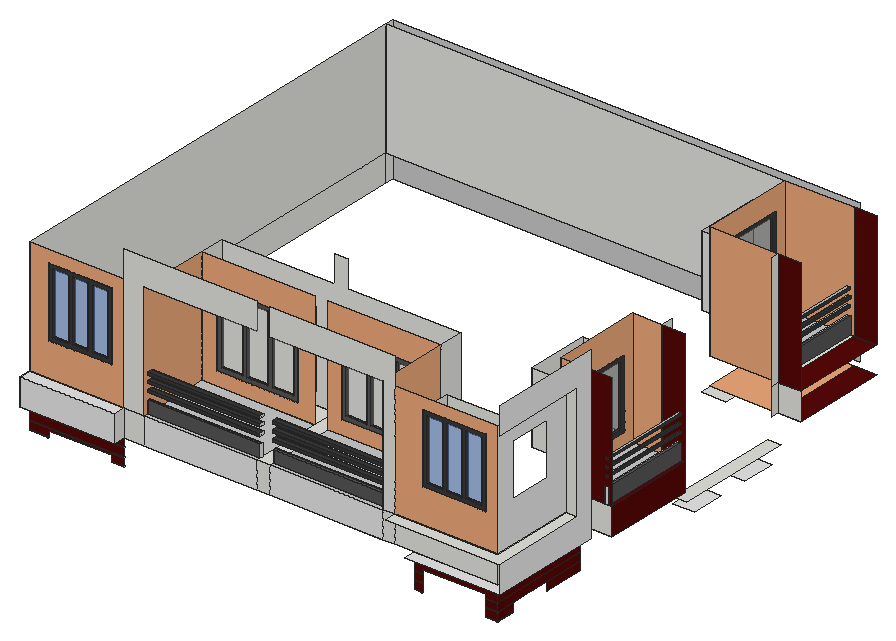
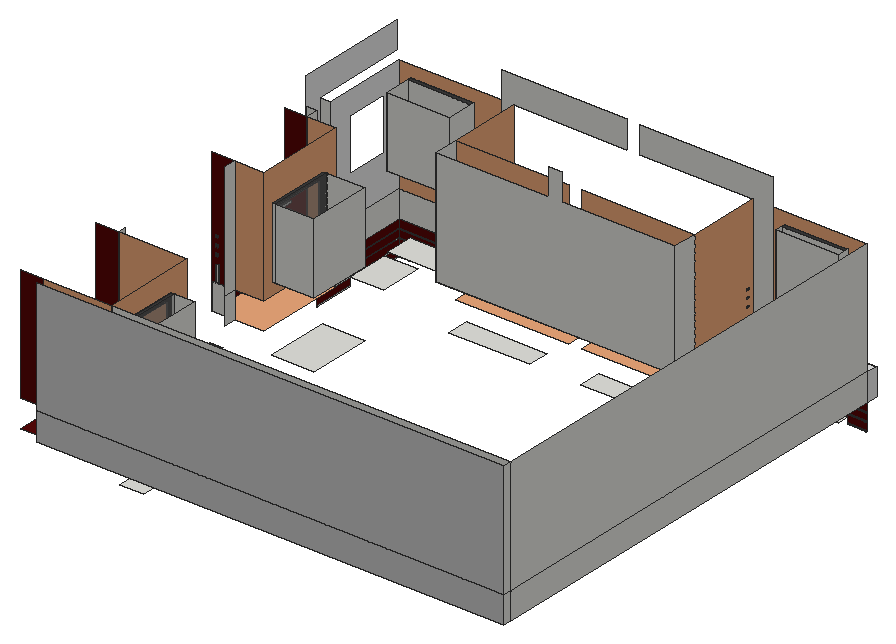
# SketchUp Ruby script. Lengths in inches.
U = 1.inch
M = Sketchup.active_model
def pt(a) = Geom::Point3d.new(a.map { |v| v * U })
def face(e, loops, mat)
  f = e.add_face(loops[0].map { |a| pt(a) })
  loops[1..].each { |l| e.add_face(l.map { |a| pt(a) }).erase! }
  f.material = f.back_material = mat if mat
  f
end
# faces: each face lists its corners as indices into pts; further lists are holes
def faces(e, pts, list, mat = nil) = list.each { |f| face(e, (f[0].is_a?(Array) ? f : [f]).map { |l| l.map { |i| pts[i] } }, mat) }
# xy, xz, yz: faces in a plane at the given z, y or x. An outline is a flat list of corners, or four numbers for a rectangle; further outlines are holes
def ring(l) = l.size == 4 ? [[l[0], l[1]], [l[2], l[1]], [l[2], l[3]], [l[0], l[3]]] : l.each_slice(2).to_a
def flat(e, list, mat, &to3) = list.each { |f| face(e, (f[0].is_a?(Array) ? f : [f]).map { |l| ring(l).map { |u, v| to3.(u, v) } }, mat) }
def xy(e, z, list, mat = nil) = flat(e, list, mat) { |x, y| [x, y, z] }
def xz(e, y, list, mat = nil) = flat(e, list, mat) { |x, z| [x, y, z] }
def yz(e, x, list, mat = nil) = flat(e, list, mat) { |y, z| [x, y, z] }
def lines(e, pts, list) = list.each { |a, b| e.add_line(pt(pts[a]), pt(pts[b])) }
# prism: a flat outline (further loops are holes) pulled along v
def prism(e, loops, v, mat = nil)
  f = face(e, loops, mat); d = Geom::Vector3d.new(v.map { |x| x * U })
  f.pushpull(f.normal.samedirection?(d) ? d.length : -d.length)
end
def box(e, o, s, mat = nil) = prism(e, [[o, [o[0] + s[0], o[1], o[2]], [o[0] + s[0], o[1] + s[1], o[2]], [o[0], o[1] + s[1], o[2]]]], [0, 0, s[2]], mat)
def at(x, y, z, deg = 0) = Geom::Transformation.translation(pt([x, y, z])) * Geom::Transformation.rotation(ORIGIN, Z_AXIS, deg.degrees)
def axes(o, x, y, z) = Geom::Transformation.new([*x, 0, *y, 0, *z, 0, *pt(o).to_a, 1])
def part(name) = M.definitions.add(name)
# library, detail: a bought-in or finely detailed component or shape, given as its bounding box
def library(name, o, s) = part(name).tap { |d| box(d.entities, o, s) }
def detail(e, o, s) = box(e.add_group.entities, o, s)
def put(e, d, t, mat = nil) = e.add_instance(d, t).tap { |i| i.material = mat if mat }
def group(e, t, mat = nil) = e.add_group.tap { |g| g.transformation = t; g.material = mat if mat }.entities
root = M.entities
M.materials.add("Generic").color = [86, 8, 8]
M.materials.add("Generic\#1").color = [236, 168, 122]
M.materials.add("Generic\#4").color = [201, 201, 201]
M.materials.add("Generic\#5").color = [230, 230, 230]
M.materials.add("[Color M06]").color = [86, 86, 86]
M.materials.add("[Color M07]").color = [58, 58, 58]
M.materials.add("[Mirror 02]1").color = [226, 226, 226]
M.materials["[Mirror 02]1"].alpha = 0.26
M.materials.add("[Translucent Glass Blue]").color = [100, 149, 237]
M.materials["[Translucent Glass Blue]"].alpha = 0.5
M.materials.add("[Translucent Glass Gray]").color = [127, 127, 127]
M.materials["[Translucent Glass Gray]"].alpha = 0.35
c1 = library("Tlon Light 450 Ceiling 152 006",[-8.86,-8.86,-3.78],[17.72,17.72,3.56])
c2 = part("Group\#5")
xy(c2.entities,0,[[0,0,6,92.0625]],"[Color M07]")
xy(c2.entities,6.58,[[3,6.58,6,85.48]],"[Color M07]")
xy(c2.entities,96.73,[[3,6.58,6,85.48]],"[Color M07]")
xy(c2.entities,103.3125,[[0,0,6,92.0625]],"[Color M07]")
xz(c2.entities,0,[[0,0,6,103.3125]],"[Color M07]")
xz(c2.entities,6.58,[[3,6.58,6,96.73]],"[Color M07]")
xz(c2.entities,85.48,[[3,6.58,6,96.73]],"[Color M07]")
xz(c2.entities,92.0625,[[0,0,6,103.3125]],"[Color M07]")
yz(c2.entities,0,[[0,0,92.0625,103.3125]],"[Translucent Glass Gray]")
yz(c2.entities,3,[[6.58,6.58,85.48,96.73]],"[Translucent Glass Gray]")
yz(c2.entities,6,[[[0,0,92.0625,103.3125],[6.58,6.58,85.48,96.73]]],"[Color M07]")
c3 = part("Group\#4")
xy(c3.entities,0,[[0,0,117.75,6]],"[Color M06]")
xy(c3.entities,6.37,[[6.37,0,37.125,3],[43.5,0,74.25,3],[80.625,0,111.38,3]],"[Color M06]")
xy(c3.entities,103.75,[[6.37,0,37.125,3],[43.5,0,74.25,3],[80.625,0,111.38,3]],"[Color M06]")
xy(c3.entities,110.125,[[0,0,117.75,6]],"[Color M06]")
xz(c3.entities,0,[[[0,0,117.75,110.125],[6.37,6.37,37.125,103.75],[80.625,6.37,111.38,103.75],[43.5,6.37,74.25,103.75]]],"[Color M06]")
xz(c3.entities,3,[[6.37,6.37,37.125,103.75],[43.5,6.37,74.25,103.75],[80.625,6.37,111.38,103.75]],"[Mirror 02]1")
xz(c3.entities,6,[[0,0,117.75,110.125]])
yz(c3.entities,0,[[0,0,6,110.125]],"[Color M06]")
yz(c3.entities,6.37,[[0,6.37,3,103.75]],"[Color M06]")
yz(c3.entities,37.125,[[0,6.37,3,103.75]],"[Color M06]")
yz(c3.entities,43.5,[[0,6.37,3,103.75]],"[Color M06]")
yz(c3.entities,74.25,[[0,6.37,3,103.75]],"[Color M06]")
yz(c3.entities,80.625,[[0,6.37,3,103.75]],"[Color M06]")
yz(c3.entities,111.38,[[0,6.37,3,103.75]],"[Color M06]")
yz(c3.entities,117.75,[[0,0,6,110.125]],"[Color M06]")
c4 = part("Group\#2")
xy(c4.entities,0,[[0,0,91.6875,6]],"[Color M07]")
xy(c4.entities,6.1,[[6.1,0,28.53,3],[34.63,0,57.06,3],[63.16,0,85.59,3]],"[Color M07]")
xy(c4.entities,95.34,[[6.1,0,28.53,3],[34.63,0,57.06,3],[63.16,0,85.59,3]],"[Color M07]")
xy(c4.entities,101.4375,[[0,0,91.6875,6]],"[Color M07]")
xz(c4.entities,0,[[[0,0,91.6875,101.4375],[34.63,6.1,57.06,95.34],[63.16,6.1,85.59,95.34],[6.1,6.1,28.53,95.34]]],"[Color M07]")
xz(c4.entities,3,[[6.1,6.1,28.53,95.34],[34.63,6.1,57.06,95.34],[63.16,6.1,85.59,95.34]],"[Translucent Glass Blue]")
xz(c4.entities,6,[[0,0,91.6875,101.4375]])
yz(c4.entities,0,[[0,0,6,101.4375]],"[Color M07]")
yz(c4.entities,6.1,[[0,6.1,3,95.34]],"[Color M07]")
yz(c4.entities,28.53,[[0,6.1,3,95.34]],"[Color M07]")
yz(c4.entities,34.63,[[0,6.1,3,95.34]],"[Color M07]")
yz(c4.entities,57.06,[[0,6.1,3,95.34]],"[Color M07]")
yz(c4.entities,63.16,[[0,6.1,3,95.34]],"[Color M07]")
yz(c4.entities,85.59,[[0,6.1,3,95.34]],"[Color M07]")
yz(c4.entities,91.6875,[[0,0,6,101.4375]],"[Color M07]")
xy(root,741.1,[[577.6875,113.625,589.83,113.92],[681.51,113.625,698.4375,113.92],[698.14,113.92,698.4375,141.33]])
xy(root,741.23,[[698.14,204.02,698.4375,263.625]])
xy(root,742.1,[[577.6875,113.625,589.83,113.92],[681.51,113.625,698.14,113.92]])
xy(root,742.11,[[698.14,113.625,698.4375,141.33]])
xy(root,742.23,[[698.14,204.02,698.4375,263.625]])
xy(root,743.55,[[685.875,449.87,717.1875,498.18],[685.875,541.87,717.1875,590.18]],"Generic\#5")
xy(root,751.9375,[[16.6875,113.625,44.83,113.625,44.83,113.93,16.6875,113.92],[136.51,113.625,154.5,113.625,154.5,113.92,136.51,113.93]])
xy(root,752.29,[[594.5625,306.16,656.0625,398.23]])
xy(root,752.9375,[[16.6875,113.625,16.6875,113.92,44.83,113.93,44.83,113.625],[136.51,113.625,136.51,113.93,154.5,113.92,154.5,113.625]])
xy(root,753.05,[[577.6875,113.625,589.83,113.625,589.83,113.93,577.6875,113.92],[681.51,113.625,698.4375,113.625,698.4375,113.92,698.14,113.92,681.51,113.93],[698.14,113.92,698.4375,141.33]])
xy(root,753.13,[[698.14,204.02,698.4375,263.625]])
xy(root,754.05,[[577.6875,113.625,577.6875,113.92,589.83,113.93,589.83,113.625],[681.51,113.625,681.51,113.93,698.14,113.92,698.4375,113.92,698.4375,113.625],[698.14,113.92,698.4375,141.33]])
xy(root,754.13,[[698.14,204.02,698.4375,263.625]])
xy(root,754.24,[[648.625,141.33,698.4375,204.02]])
xy(root,755.96,[[563.75,654.65,598.75,746.71]])
xy(root,761.05,[[44.83,113.625,136.51,130.0625]])
xy(root,762.91,[[698.4375,434.68,717.1875,606.05]])
xy(root,764.4375,[[16.6875,113.625,154.5,113.92]])
xy(root,764.99,[[577.6875,113.625,589.83,113.625,589.83,113.93,577.6875,113.92],[681.51,113.625,698.4375,113.625,698.4375,113.92,681.51,113.93]])
xy(root,765.04,[[698.14,113.92,698.4375,263.625]])
xy(root,765.4375,[[16.6875,113.625,154.5,113.92]])
xy(root,765.99,[[577.6875,113.625,577.6875,113.92,589.83,113.93,589.83,113.625],[681.51,113.625,681.51,113.93,698.14,113.92,698.14,113.625]])
xy(root,766.04,[[698.14,113.625,698.4375,263.625]])
xy(root,766.34,[[205.11,219.4375,322.86,251.5625],[397.99,219.4375,515.74,251.5625]])
xy(root,771.36,[[589.83,113.625,681.51,156.125]])
xy(root,776.9375,[[16.6875,113.625,154.5,113.92],[577.6875,113.625,698.4375,113.92],[698.14,113.92,698.4375,263.625]])
xy(root,777.9375,[[16.6875,113.625,154.5,113.92],[577.6875,113.625,698.4375,113.92],[698.14,113.92,698.4375,263.625]])
xy(root,789.9375,[[698.4375,624.8125,731.4375,762.8125]],"Generic")
xy(root,789.9375,[[183.5625,113.625,347.9375,219.4375],[367.1875,113.625,531.5625,219.4375],[656.0625,281.625,731.4375,413.625],[598.75,624.8125,698.4375,762.8125]],"Generic\#1")
xy(root,789.9375,[[16.6875,96.5625,154.5,113.625],[577.6875,96.5625,577.6875,113.625,698.4375,113.625,698.4375,263.625,715.125,263.625,715.125,96.5625]],"Generic\#5")
xy(root,829.25,[[549.5625,96.5625,715.125,96.5625,715.125,238.3125,698.4375,238.3125,698.4375,113.625,549.5625,113.625],[347.9375,113.625,367.1875,255],[183.5625,119.625,347.9375,123.625],[367.1875,119.625,531.5625,123.625],[183.5625,219.4375,347.9375,255],
  [367.1875,219.4375,531.5625,255],[721.25,281.625,726.125,413.625],[689.125,624.8125,693.625,762.8125],[693.625,624.8125,698.4375,762.8125]])
xy(root,829.25,[[726.125,281.625,731.4375,413.625],[698.4375,624.8125,731.4375,762.8125]],"Generic")
xy(root,829.25,[[183.5625,113.625,347.9375,119.625],[367.1875,113.625,531.5625,119.625],[183.5625,123.625,347.9375,219.4375],[367.1875,123.625,531.5625,219.4375],[656.0625,281.625,721.25,413.625],
  [598.75,624.8125,689.125,762.8125]],"Generic\#4")
xy(root,829.25,[[16.6875,96.5625,154.5,113.625]],"Generic\#5")
xy(root,847.25,[[183.5625,119.625,347.9375,123.625],[367.1875,119.625,531.5625,123.625]],"[Color M06]")
xy(root,848.17,[[594.5625,306.16,656.0625,398.23]])
xy(root,849.15,[[205.11,219.4375,322.86,251.5625],[386.36,219.4375,504.11,251.5625]])
xy(root,853.25,[[721.25,281.625,726.125,413.625],[689.125,624.8125,693.625,762.8125]],"[Color M06]")
xy(root,857.82,[[367.1875,118.5,531.5625,125.9375]],"[Color M07]")
xy(root,857.85,[[183.5625,118.5,347.9375,125.9375]],"[Color M07]")
xy(root,861.63,[[367.1875,118.5,531.5625,125.9375]],"[Color M07]")
xy(root,861.67,[[183.5625,118.5,347.9375,125.9375]],"[Color M07]")
xy(root,863.09,[[563.75,654.65,598.75,746.71]])
xy(root,864.125,[[688.99,624.8125,693.18,762.8125]],"[Color M07]")
xy(root,864.35,[[722.32,281.625,725.7,413.625]],"[Color M07]")
xy(root,867.4375,[[688.99,624.8125,693.18,762.8125]],"[Color M07]")
xy(root,867.48,[[722.32,281.625,725.7,413.625]],"[Color M07]")
xy(root,869.58,[[367.1875,118.5,531.5625,125.9375]],"[Color M07]")
xy(root,869.85,[[183.5625,118.5,347.9375,125.9375]],"[Color M07]")
xy(root,873.39,[[367.1875,118.5,531.5625,125.9375]],"[Color M07]")
xy(root,873.67,[[183.5625,118.5,347.9375,125.9375]],"[Color M07]")
xy(root,876.125,[[689.37,624.8125,693.56,762.8125]],"[Color M07]")
xy(root,876.22,[[722.32,281.625,725.7,413.625]],"[Color M07]")
xy(root,878.93,[[44.83,113.625,136.51,130.0625],[589.83,113.625,681.51,158.0625]])
xy(root,879.34,[[722.32,281.625,725.7,413.625]],"[Color M07]")
xy(root,879.4375,[[689.37,624.8125,693.56,762.8125]],"[Color M07]")
xy(root,880.92,[[183.5625,118.5,347.9375,125.9375]],"[Color M07]")
xy(root,881.34,[[367.1875,118.5,531.5625,125.9375]],"[Color M07]")
xy(root,884.73,[[183.5625,118.5,347.9375,125.9375]],"[Color M07]")
xy(root,885.15,[[367.1875,118.5,531.5625,125.9375]],"[Color M07]")
xy(root,888.125,[[688.93,624.8125,693.12,762.8125]],"[Color M07]")
xy(root,888.22,[[722.32,281.625,725.7,413.625]],"[Color M07]")
xz(root,96.5625,[[16.6875,789.9375,154.5,829.25]],"Generic\#5")
xz(root,113.625,[[16.6875,789.9375,154.5,829.25],[154.5,789.9375,183.4375,829.25],[347.9375,789.9375,367.1875,829.25],[531.6875,789.9375,549.5625,829.25],[549.5625,789.9375,698.4375,829.25],
  [154.5,829.25,154.5,1036.5625,347.9375,1036.5625,347.9375,997.25,183.4375,997.25,183.4375,829.25],[183.4375,829.25,183.5625,997.25],[531.6875,829.25,531.6875,997.25,367.1875,997.25,367.1875,1036.5625,549.5625,1036.5625,549.5625,829.25],[531.5625,829.25,531.6875,997.25]])
xz(root,113.625,[[577.6875,742.1,589.83,753.05],[681.51,742.1,698.14,742.1,698.14,742.11,698.4375,742.11,698.4375,753.05,681.51,753.05],[16.6875,752.9375,44.83,752.9375,44.83,761.05,136.51,761.05,136.51,752.9375,154.5,752.9375,154.5,764.4375,16.6875,764.4375],[577.6875,754.05,589.83,764.99],[681.51,754.05,698.4375,764.99],
  [16.6875,765.4375,154.5,776.9375],[577.6875,765.99,589.83,765.99,589.83,771.36,681.51,771.36,681.51,765.99,698.14,765.99,698.14,766.04,698.4375,766.04,698.4375,776.9375,577.6875,776.9375],[16.6875,777.9375,154.5,789.9375],[577.6875,777.9375,698.4375,789.9375]],"Generic")
xz(root,113.625,[[[16.6875,829.25,154.5,997.25],[44.83,878.93,136.51,980.36]],[[549.5625,829.25,698.4375,997.25],[589.83,878.93,681.51,980.36]]],"Generic\#1")
xz(root,113.625,[[183.4375,789.9375,347.9375,829.25],[367.1875,789.9375,531.6875,829.25]],"Generic\#5")
xz(root,113.92,[[577.6875,741.1,589.83,742.1],[681.51,741.1,698.14,742.1],[16.6875,764.4375,154.5,765.4375],[16.6875,776.9375,154.5,777.9375],[577.6875,776.9375,698.14,777.9375]])
xz(root,118.5,[[367.1875,857.82,531.5625,861.63],[183.5625,857.85,347.9375,861.67],[367.1875,869.58,531.5625,873.39],[183.5625,869.85,347.9375,873.67],[183.5625,880.92,347.9375,884.73],
  [367.1875,881.34,531.5625,885.15]],"[Color M07]")
xz(root,119.625,[[183.5625,829.25,347.9375,847.25],[367.1875,829.25,531.5625,847.25]],"[Color M06]")
xz(root,123.625,[[183.5625,829.25,347.9375,847.25],[367.1875,829.25,531.5625,847.25]])
xz(root,125.9375,[[367.1875,857.82,531.5625,861.63],[183.5625,857.85,347.9375,861.67],[367.1875,869.58,531.5625,873.39],[183.5625,869.85,347.9375,873.67],[183.5625,880.92,347.9375,884.73],
  [367.1875,881.34,531.5625,885.15]])
xz(root,130.0625,[[44.83,878.93,136.51,980.36]])
xz(root,158.0625,[[589.83,878.93,681.51,980.36]])
xz(root,219.4375,[[[183.5625,829.25,347.9375,997.25],[205.11,849.15,322.86,959.27]],[[367.1875,829.25,531.5625,997.25],[386.36,849.15,504.11,959.27]]],"Generic\#1")
xz(root,238.3125,[[698.4375,829.25,715.125,997.25]])
xz(root,251.5625,[[205.11,849.15,322.86,959.27],[386.36,849.15,504.11,959.27]])
xz(root,255,[[183.5625,829.25,531.5625,829.25,531.5625,997.25,367.1875,997.25,367.1875,1036.5625,347.9375,1036.5625,347.9375,997.25,183.5625,997.25]])
xz(root,263.625,[[698.14,741.23,698.4375,742.23],[698.14,753.13,698.4375,754.13],[698.14,765.04,698.4375,766.04],[698.14,776.9375,698.4375,777.9375],[698.4375,789.9375,715.125,829.25],
  [698.4375,829.25,715.125,997.25]])
xz(root,281.625,[[698.4375,789.9375,731.4375,829.25],[721.25,829.25,726.125,853.25]])
xz(root,281.625,[[[698.4375,829.25,698.4375,997.25,731.4375,997.25,731.4375,829.25,726.125,829.25,726.125,853.25,721.25,853.25,721.25,829.25],[722.32,888.22,725.7,891.34],[722.32,876.22,725.7,879.34],[722.32,864.35,725.7,867.48]]],"Generic")
xz(root,281.625,[[656.0625,829.25,698.4375,997.25]],"Generic\#1")
xz(root,306.16,[[594.5625,848.17,656.0625,951.48]])
xz(root,398.23,[[594.5625,848.17,656.0625,951.48]])
xz(root,413.625,[[698.4375,789.9375,731.4375,829.25],[721.25,829.25,726.125,853.25],[722.32,864.35,725.7,867.48],[722.32,876.22,725.7,879.34],[722.32,888.22,725.7,891.34]])
xz(root,413.625,[[[698.4375,829.25,721.25,829.25,721.25,853.25,726.125,853.25,726.125,829.25,731.4375,829.25,731.4375,997.25,698.4375,997.25],[722.32,864.35,725.7,867.48],[722.32,876.22,725.7,879.34],[722.32,888.22,725.7,891.34]]],"Generic")
xz(root,413.625,[[656.0625,829.25,698.4375,997.25]],"Generic\#1")
xz(root,624.8125,[[698.4375,789.9375,731.4375,829.25],[689.125,829.25,693.625,853.25]])
xz(root,624.8125,[[698.4375,829.25,731.4375,997.25]],"Generic")
xz(root,624.8125,[[[598.75,829.25,598.75,997.25,698.4375,997.25,698.4375,829.25,693.625,829.25,693.625,853.25,689.125,853.25,689.125,829.25],[688.93,888.125,693.12,891.4375],[689.37,876.125,693.56,879.4375],[688.99,864.125,693.18,867.4375]]],"Generic\#1")
xz(root,654.65,[[563.75,863.09,598.75,966.4]])
xz(root,746.71,[[563.75,863.09,598.75,966.4]])
xz(root,762.8125,[[16.6875,829.25,598.75,997.25],[689.125,829.25,693.625,853.25],[688.99,864.125,693.18,867.4375],[689.37,876.125,693.56,879.4375],[688.93,888.125,693.12,891.4375]])
xz(root,762.8125,[[698.4375,829.25,731.4375,997.25]],"Generic")
xz(root,762.8125,[[[598.75,829.25,689.125,829.25,689.125,853.25,693.625,853.25,693.625,829.25,698.4375,829.25,698.4375,997.25,598.75,997.25],[688.99,864.125,693.18,867.4375],[689.37,876.125,693.56,879.4375],[688.93,888.125,693.12,891.4375]]],"Generic\#1")
xz(root,774.8125,[[16.6875,789.9375,698.4375,829.25],[16.6875,829.25,698.4375,997.25]],"Generic\#4")
yz(root,16.6875,[[113.625,789.9375,762.8125,829.25],[762.8125,789.9375,774.8125,829.25],[113.625,829.25,762.8125,997.25],[762.8125,829.25,774.8125,997.25]])
yz(root,16.6875,[[96.5625,789.9375,113.625,829.25]],"Generic\#5")
yz(root,44.83,[[113.625,878.93,130.0625,980.36]])
yz(root,136.51,[[113.625,878.93,130.0625,980.36]])
yz(root,154.5,[[113.625,751.9375,113.92,752.9375],[113.625,764.4375,113.92,765.4375],[113.625,776.9375,113.92,777.9375],[96.5625,789.9375,113.625,829.25]])
yz(root,183.5625,[[119.625,829.25,123.625,847.25],[219.4375,829.25,255,997.25]])
yz(root,183.5625,[[[113.625,829.25,119.625,829.25,119.625,847.25,123.625,847.25,123.625,829.25,219.4375,829.25,219.4375,997.25,113.625,997.25],[118.5,880.92,125.9375,884.73],[118.5,869.85,125.9375,873.67],[118.5,857.85,125.9375,861.67]]],"Generic\#1")
yz(root,205.11,[[219.4375,849.15,251.5625,959.27]])
yz(root,322.86,[[219.4375,849.15,251.5625,959.27]])
yz(root,347.9375,[[119.625,829.25,123.625,847.25],[118.5,857.85,125.9375,861.67],[118.5,869.85,125.9375,873.67],[118.5,880.92,125.9375,884.73]])
yz(root,367.1875,[[119.625,829.25,123.625,847.25]])
yz(root,386.36,[[219.4375,849.15,251.5625,959.27]])
yz(root,504.11,[[219.4375,849.15,251.5625,959.27]])
yz(root,531.5625,[[119.625,829.25,123.625,847.25],[219.4375,829.25,255,997.25],[118.5,857.82,125.9375,861.63],[118.5,869.58,125.9375,873.39],[118.5,881.34,125.9375,885.15]])
yz(root,531.5625,[[[113.625,829.25,113.625,997.25,219.4375,997.25,219.4375,829.25,123.625,829.25,123.625,847.25,119.625,847.25,119.625,829.25],[118.5,881.34,125.9375,885.15],[118.5,869.58,125.9375,873.39],[118.5,857.82,125.9375,861.63]]],"Generic\#1")
yz(root,563.75,[[654.65,863.09,746.71,966.4]])
yz(root,577.6875,[[113.625,741.1,113.92,742.1],[113.625,753.05,113.92,754.05],[113.625,764.99,113.92,765.99],[113.625,776.9375,113.92,777.9375]])
yz(root,589.83,[[113.625,878.93,158.0625,980.36]])
yz(root,594.5625,[[306.16,848.17,398.23,951.48]])
yz(root,598.75,[[[624.8125,829.25,762.8125,997.25],[654.65,863.09,746.71,966.4]]],"Generic\#1")
yz(root,656.0625,[[[281.625,829.25,413.625,997.25],[306.16,848.17,398.23,951.48]]],"Generic\#1")
yz(root,681.51,[[113.625,878.93,158.0625,980.36]])
yz(root,688.93,[[624.8125,888.125,762.8125,891.4375]])
yz(root,688.99,[[624.8125,864.125,762.8125,867.4375]])
yz(root,689.125,[[624.8125,829.25,762.8125,853.25]])
yz(root,689.37,[[624.8125,876.125,762.8125,879.4375]])
yz(root,693.12,[[624.8125,888.125,762.8125,891.4375]],"[Color M07]")
yz(root,693.18,[[624.8125,864.125,762.8125,867.4375]],"[Color M07]")
yz(root,693.56,[[624.8125,876.125,762.8125,879.4375]],"[Color M07]")
yz(root,693.625,[[624.8125,829.25,762.8125,853.25]],"[Color M06]")
yz(root,698.14,[[113.92,741.1,141.33,741.1,141.33,742.11,113.625,742.11,113.625,742.1,113.92,742.1],[204.02,741.23,263.625,742.23],[113.92,753.05,141.33,754.05],[204.02,753.13,263.625,754.13],[113.92,765.04,263.625,765.04,263.625,766.04,113.625,766.04,113.625,765.99,113.92,765.99],
  [113.92,776.9375,263.625,777.9375]])
yz(root,698.4375,[[113.625,789.9375,263.625,829.25],[263.625,789.9375,281.625,829.25],[413.625,789.9375,431.625,829.25],[612.8125,789.9375,624.8125,829.25],[263.625,829.25,281.625,997.25],
  [413.625,829.25,431.625,997.25],[612.8125,829.25,624.8125,997.25]])
yz(root,698.4375,[[113.625,742.11,141.33,753.05],[204.02,742.23,263.625,753.13],[113.625,754.05,141.33,754.05,141.33,754.24,204.02,754.24,204.02,754.13,263.625,754.13,263.625,765.04,113.92,765.04,113.92,764.99,113.625,764.99],[113.625,766.04,263.625,776.9375],[113.625,777.9375,263.625,789.9375]],"Generic")
yz(root,698.4375,[[[113.625,829.25,238.3125,997.25],[141.33,889.17,204.02,964.8]]],"Generic\#5")
yz(root,715.125,[[96.5625,789.9375,263.625,789.9375,263.625,1036.5625,96.5625,1036.5625,96.5625,997.25,238.3125,997.25,238.3125,829.25,96.5625,829.25]],"Generic\#5")
yz(root,721.25,[[281.625,829.25,413.625,853.25]])
yz(root,722.32,[[281.625,864.35,413.625,867.48],[281.625,876.22,413.625,879.34],[281.625,888.22,413.625,891.34]])
yz(root,725.7,[[281.625,864.35,413.625,867.48],[281.625,876.22,413.625,879.34],[281.625,888.22,413.625,891.34]],"[Color M07]")
yz(root,726.125,[[281.625,829.25,413.625,853.25]],"[Color M06]")
yz(root,731.4375,[[281.625,789.9375,413.625,829.25]],"Generic")
p = [[16.6875,113.92,751.9375],[44.83,113.93,751.9375],[44.83,113.93,752.9375],[16.6875,113.92,752.9375],[154.5,113.92,751.9375],[154.5,113.92,752.9375],
  [136.51,113.93,752.9375],[136.51,113.93,751.9375],[589.83,113.93,753.05],[589.83,113.93,754.05],[577.6875,113.92,754.05],[577.6875,113.92,753.05],
  [698.14,113.92,754.05],[681.51,113.93,754.05],[681.51,113.93,753.05],[698.14,113.92,753.05],[577.6875,113.92,764.99],[589.83,113.93,764.99],
  [589.83,113.93,765.99],[577.6875,113.92,765.99],[681.51,113.93,765.99],[681.51,113.93,764.99],[698.4375,113.92,764.99],[698.4375,113.92,765.04],
  [698.14,113.92,765.04],[698.14,113.92,765.99],[531.5625,121.625,859.25],[367.1875,121.625,859.25],[531.5625,121.625,871.25],[367.1875,121.625,871.25],
  [531.5625,121.625,883.25],[367.1875,121.625,883.25],[347.9375,121.625,859.25],[183.5625,121.625,859.25],[347.9375,121.625,871.25],[183.5625,121.625,871.25],
  [347.9375,121.625,883.25],[183.5625,121.625,883.25],[691.375,762.8125,865.25],[691.375,624.8125,865.25],[691.375,762.8125,877.25],[691.375,624.8125,877.25],
  [723.6875,413.625,865.25],[723.6875,281.625,865.25],[723.6875,413.625,877.25],[723.6875,281.625,877.25],[698.4375,141.33,754.05],[698.4375,204.02,754.13]]
faces(root,p,[[0,1,2,3],[4,5,6,7],[8,9,10,11],[12,13,14,15],[16,17,18,19],[20,21,22,23,24,25]])
lines(root,p,[[26,27],[28,29],[30,31],[32,33],[34,35],[36,37],[38,39],[40,41],[42,43],[44,45],[46,47]])
put(root,c1,at(507.78,141.27,791.6))
put(root,c1,at(412.28,141.27,791.6))
put(root,c1,at(320.22,141.27,791.6))
put(root,c1,at(220.41,141.27,791.6))
put(root,c2,at(650.0625,306.16,848.17))
put(root,c3,at(386.36,219.4375,849.15))
put(root,c3,at(205.11,219.4375,849.15))
put(root,c2,at(592.75,654.65,863.09))
put(root,c4,at(589.83,113.625,878.93))
put(root,c4,at(44.83,113.625,878.93))
